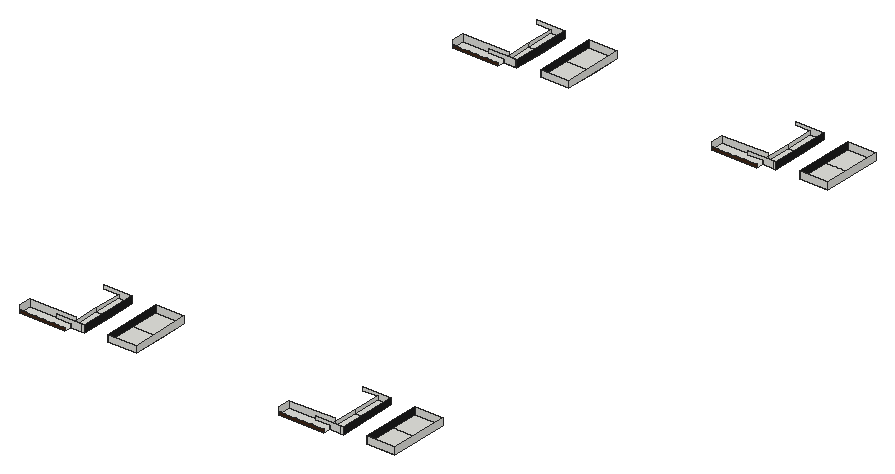
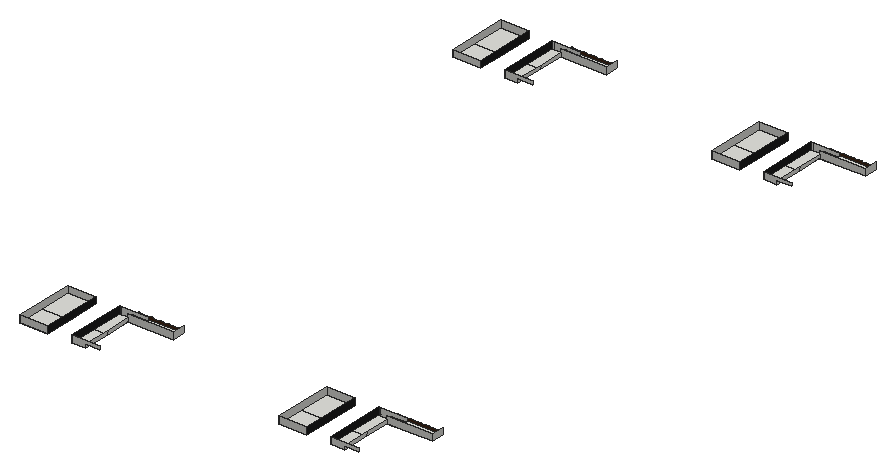
# SketchUp Ruby script. Lengths in inches.
U = 1.inch
M = Sketchup.active_model
def pt(a) = Geom::Point3d.new(a.map { |v| v * U })
def face(e, loops, mat)
  f = e.add_face(loops[0].map { |a| pt(a) })
  loops[1..].each { |l| e.add_face(l.map { |a| pt(a) }).erase! }
  f.material = f.back_material = mat if mat
  f
end
# faces: each face lists its corners as indices into pts; further lists are holes
def faces(e, pts, list, mat = nil) = list.each { |f| face(e, (f[0].is_a?(Array) ? f : [f]).map { |l| l.map { |i| pts[i] } }, mat) }
# xy, xz, yz: faces in a plane at the given z, y or x. An outline is a flat list of corners, or four numbers for a rectangle; further outlines are holes
def ring(l) = l.size == 4 ? [[l[0], l[1]], [l[2], l[1]], [l[2], l[3]], [l[0], l[3]]] : l.each_slice(2).to_a
def flat(e, list, mat, &to3) = list.each { |f| face(e, (f[0].is_a?(Array) ? f : [f]).map { |l| ring(l).map { |u, v| to3.(u, v) } }, mat) }
def xy(e, z, list, mat = nil) = flat(e, list, mat) { |x, y| [x, y, z] }
def xz(e, y, list, mat = nil) = flat(e, list, mat) { |x, z| [x, y, z] }
def yz(e, x, list, mat = nil) = flat(e, list, mat) { |y, z| [x, y, z] }
def lines(e, pts, list) = list.each { |a, b| e.add_line(pt(pts[a]), pt(pts[b])) }
# prism: a flat outline (further loops are holes) pulled along v
def prism(e, loops, v, mat = nil)
  f = face(e, loops, mat); d = Geom::Vector3d.new(v.map { |x| x * U })
  f.pushpull(f.normal.samedirection?(d) ? d.length : -d.length)
end
def box(e, o, s, mat = nil) = prism(e, [[o, [o[0] + s[0], o[1], o[2]], [o[0] + s[0], o[1] + s[1], o[2]], [o[0], o[1] + s[1], o[2]]]], [0, 0, s[2]], mat)
def at(x, y, z, deg = 0) = Geom::Transformation.translation(pt([x, y, z])) * Geom::Transformation.rotation(ORIGIN, Z_AXIS, deg.degrees)
def axes(o, x, y, z) = Geom::Transformation.new([*x, 0, *y, 0, *z, 0, *pt(o).to_a, 1])
def part(name) = M.definitions.add(name)
# library, detail: a bought-in or finely detailed component or shape, given as its bounding box
def library(name, o, s) = part(name).tap { |d| box(d.entities, o, s) }
def detail(e, o, s) = box(e.add_group.entities, o, s)
def put(e, d, t, mat = nil) = e.add_instance(d, t).tap { |i| i.material = mat if mat }
def group(e, t, mat = nil) = e.add_group.tap { |g| g.transformation = t; g.material = mat if mat }.entities
root = M.entities
M.materials.add("[Color M08]").color = [30, 30, 30]
M.materials.add("[Wood Veneer 01]").color = [66, 38, 20]
xy(root,230.89,[[252.78,566.68,406.85,611.02],[1131.53,566.68,1285.6,611.02],[252.78,2402.3,406.85,2446.65],[1131.53,2402.3,1285.6,2446.65]])
xy(root,231,[[406.85,589.83,453.7,697.21],[534.46,589.83,629.77,697.21],[1285.6,589.83,1332.45,697.21],[1413.21,589.83,1508.52,697.21],[406.85,697.21,453.7,792.52],
  [534.46,697.21,629.77,792.52],[1285.6,697.21,1332.45,792.52],[1413.21,697.21,1508.52,792.52],[406.85,2425.46,453.7,2532.83],[534.46,2425.46,629.77,2532.83],
  [1285.6,2425.46,1332.45,2532.83],[1413.21,2425.46,1508.52,2532.83],[406.85,2532.83,453.7,2628.15],[534.46,2532.83,629.77,2628.15],[1285.6,2532.83,1332.45,2628.15],
  [1413.21,2532.83,1508.52,2628.15]])
xz(root,566.68,[[252.78,230.89,406.85,230.89,406.85,240.89,405.02,240.1,404.46,239.96,403.9375,239.81,403.25,239.53,402.7,239.49,401.98,239.42,401.18,239.28,400.41,239.15,399.78,238.9,398.39,238.9,397.63,238.89,396.95,238.89,396.27,238.88,395.73,238.875,394.97,238.86,394.23,238.83,393.66,238.8,393.08,238.74,392.42,238.6,391.85,238.51,391.32,238.33,390.63,238.08,389.95,237.84,389.26,237.5625,388.66,237.47,387.98,237.4,387.25,237.42,386.68,237.45,386.09,237.51,385.49,237.59,384.95,237.71,384.12,238,383.41,238.33,382.86,238.57,382.36,238.86,381.84,238.96,381.15,239.02,380.47,239.125,379.73,239.04,379.16,238.66,378.57,238.61,377.91,238.55,377.39,238.27,376.71,238.18,376.03,238.18,375.36,238.11,374.83,238.15,374.01,238.19,373.4375,238.26,372.87,238.48,372.21,238.56,371.64,238.67,371.12,239.01,370.4375,239.18,369.8125,239.5,369.05,239.65,368.4375,239.8,367.68,239.96,367.03,240.23,366.45,240.27,365.8,240.43,365.23,240.43,364.65,240.42,364.125,240.41,363.43,240.4,362.74,240.37,362.05,240.33,361.37,240.27,360.69,240.17,360.07,239.97,359.42,239.75,358.68,239.375,357.89,239.08,357.01,238.72,356.26,238.46,355.04,238.14,353.92,237.88,353.27,237.87,352.4,237.74,351.69,237.79,350.92,237.86,350.29,238.15,349.52,238.19,348.9,238.25,348.14,238.45,347.45,238.62,342.56,238.62,342,238.625,341.14,238.625,340.45,238.63,339.83,238.64,339.05,238.65,338.38,238.66,337.69,238.6875,337.02,238.73,336.54,238.78,335.66,238.93,334.89,239.07,334.34,239.16,333.49,239.44,332.82,239.56,332.21,239.72,331.48,239.7,330.92,239.69,330.33,239.65,329.71,239.6,329.22,239.54,328.41,239.31,327.41,239.22,326.83,239.12,326.1875,238.76,325.55,238.51,324.99,238.375,324.55,238.02,323.85,237.74,323.23,237.43,322.38,237.22,321.7,236.98,321.09,237.01,320.4,237.04,319.64,237.11,318.95,237.2,318.42,237.33,317.75,237.68,316.8125,237.96,316.25,238.28,315.47,238.43,314.69,238.78,314.02,238.79,313.48,238.8,312.72,238.83,311.97,238.875,311.4,238.94,310.82,239.04,310.16,239.29,309.58,239.53,309.05,239.7,308.36,239.92,307.73,240.11,306.95,240.27,306.33,240.25,305.625,240.23,304.86,240.19,304.1875,240.12,303.53,240.03,302.89,239.85,302.34,239.52,301.78,239.35,301.19,239.18,300.68,238.86,299.99,238.72,299.17,238.59,298.66,238.34,293.09,238.34,292.41,238.33,291.18,238.33,290.46,238.32,289.61,238.3,288.98,238.28,288.23,238.26,287.6,238.15,286.84,238.13,286.29,238.1,285.4375,237.98,284.82,237.94,284.06,237.89,283.39,237.65,282.08,237.65,281.39,237.66,280.64,237.67,280.04,237.68,279.43,237.71,278.72,237.76,278.03,237.82,277.37,237.9,276.43,238.21,275.96,238.31,275.05,238.43,274.4,238.74,273.82,239.11,273.24,239.38,272.78,239.71,272.08,240.11,271.39,240.09,270.73,240.05,270.14,239.99,269.41,239.88,268.86,239.69,268.28,239.55,267.72,238.9375,267.19,238.77,266.45,238.79,265.58,238.8,265.07,238.82,264.03,238.92,263.34,238.93,262.64,238.94,261.94,238.97,261.26,239.03,260.57,239.09,259.79,239.19,259.28,239.52,258.72,239.64,258.27,239.86,257.48,240.2,256.88,240.59,256.34,240.85,255.32,241.55,254.05,241.69,252.84,241.52,252.78,241.52],[1131.53,230.89,1285.6,230.89,1285.6,240.89,1283.77,240.1,1283.21,239.96,1282.6875,239.81,1282,239.53,1281.45,239.49,1280.73,239.42,1279.93,239.28,1279.16,239.15,1278.53,238.9,1277.14,238.9,1276.38,238.89,1275.7,238.89,1275.02,238.88,1274.48,238.875,1273.72,238.86,1272.98,238.83,1272.41,238.8,1271.83,238.74,1271.17,238.6,1270.6,238.51,1270.07,238.33,1269.38,238.08,1268.7,237.84,1268.01,237.5625,1267.41,237.47,1266.73,237.4,1266,237.42,1265.43,237.45,1264.84,237.51,1264.24,237.59,1263.7,237.71,1262.87,238,1262.16,238.33,1261.61,238.57,1261.11,238.86,1260.59,238.96,1259.9,239.02,1259.22,239.125,1258.48,239.04,1257.91,238.66,1257.32,238.61,1256.66,238.55,1256.14,238.27,1255.46,238.18,1254.78,238.18,1254.11,238.11,1253.58,238.15,1252.76,238.19,1252.1875,238.26,1251.62,238.48,1250.96,238.56,1250.39,238.67,1249.87,239.01,1249.1875,239.18,1248.5625,239.5,1247.8,239.65,1247.1875,239.8,1246.43,239.96,1245.78,240.23,1245.2,240.27,1244.55,240.43,1243.98,240.43,1243.4,240.42,1242.875,240.41,1242.18,240.4,1241.49,240.37,1240.8,240.33,1240.12,240.27,1239.44,240.17,1238.82,239.97,1238.17,239.75,1237.43,239.375,1236.64,239.08,1235.76,238.72,1235.01,238.46,1233.79,238.14,1232.67,237.88,1232.02,237.87,1231.15,237.74,1230.44,237.79,1229.67,237.86,1229.04,238.15,1228.27,238.19,1227.65,238.25,1226.89,238.45,1226.2,238.62,1221.31,238.62,1220.75,238.625,1219.89,238.625,1219.2,238.63,1218.58,238.64,1217.8,238.65,1217.13,238.66,1216.44,238.6875,1215.77,238.73,1215.29,238.78,1214.41,238.93,1213.64,239.07,1213.09,239.16,1212.24,239.44,1211.57,239.56,1210.96,239.72,1210.23,239.7,1209.67,239.69,1209.08,239.65,1208.46,239.6,1207.97,239.54,1207.16,239.31,1206.16,239.22,1205.58,239.12,1204.9375,238.76,1204.3,238.51,1203.74,238.375,1203.3,238.02,1202.6,237.74,1201.98,237.43,1201.13,237.22,1200.45,236.98,1199.84,237.01,1199.15,237.04,1198.39,237.11,1197.7,237.2,1197.17,237.33,1196.5,237.68,1195.5625,237.96,1195,238.28,1194.22,238.43,1193.44,238.78,1192.77,238.79,1192.23,238.8,1191.47,238.83,1190.72,238.875,1190.15,238.94,1189.57,239.04,1188.91,239.29,1188.33,239.53,1187.8,239.7,1187.11,239.92,1186.48,240.11,1185.7,240.27,1185.08,240.25,1184.375,240.23,1183.61,240.19,1182.9375,240.12,1182.28,240.03,1181.64,239.85,1181.09,239.52,1180.53,239.35,1179.94,239.18,1179.43,238.86,1178.74,238.72,1177.92,238.59,1177.41,238.34,1171.84,238.34,1171.16,238.33,1169.93,238.33,1169.21,238.32,1168.36,238.3,1167.73,238.28,1166.98,238.26,1166.35,238.15,1165.59,238.13,1165.04,238.1,1164.1875,237.98,1163.57,237.94,1162.81,237.89,1162.14,237.65,1160.83,237.65,1160.14,237.66,1159.39,237.67,1158.79,237.68,1158.18,237.71,1157.47,237.76,1156.78,237.82,1156.12,237.9,1155.18,238.21,1154.71,238.31,1153.8,238.43,1153.15,238.74,1152.57,239.11,1151.99,239.38,1151.53,239.71,1150.83,240.11,1150.14,240.09,1149.48,240.05,1148.89,239.99,1148.16,239.88,1147.61,239.69,1147.03,239.55,1146.47,238.9375,1145.94,238.77,1145.2,238.79,1144.33,238.8,1143.82,238.82,1142.78,238.92,1142.09,238.93,1141.39,238.94,1140.69,238.97,1140.01,239.03,1139.32,239.09,1138.54,239.19,1138.03,239.52,1137.47,239.64,1137.02,239.86,1136.23,240.2,1135.63,240.59,1135.09,240.85,1134.07,241.55,1132.8,241.69,1131.59,241.52,1131.53,241.52]],"[Wood Veneer 01]")
xz(root,589.83,[[406.85,231,444.78,231,444.78,254.5,358.39,254.5,358.39,242.625,406.85,242.625],[444.78,231,453.7,254.5],[534.46,231,629.77,254.5],[1285.6,231,1323.53,231,1323.53,254.5,1237.14,254.5,1237.14,242.625,1285.6,242.625],[1323.53,231,1332.45,254.5],
  [1413.21,231,1508.52,254.5]])
xz(root,611.02,[[252.78,230.89,406.85,254.5],[1131.53,230.89,1285.6,254.5]])
xz(root,792.52,[[406.85,231,406.85,242.625,358.39,242.625,358.39,254.5,453.7,254.5,453.7,231],[534.46,231,629.77,254.5],[1285.6,231,1285.6,242.625,1237.14,242.625,1237.14,254.5,1332.45,254.5,1332.45,231],[1413.21,231,1508.52,254.5]])
xz(root,2402.3,[[252.78,230.89,406.85,230.89,406.85,240.89,405.02,240.1,404.46,239.96,403.9375,239.81,403.25,239.53,402.7,239.49,401.98,239.42,401.18,239.28,400.41,239.15,399.78,238.9,398.39,238.9,397.63,238.89,396.95,238.89,396.27,238.88,395.73,238.875,394.97,238.86,394.23,238.83,393.66,238.8,393.08,238.74,392.42,238.6,391.85,238.51,391.32,238.33,390.63,238.08,389.95,237.84,389.26,237.5625,388.66,237.47,387.98,237.4,387.25,237.42,386.68,237.45,386.09,237.51,385.49,237.59,384.95,237.71,384.12,238,383.41,238.33,382.86,238.57,382.36,238.86,381.84,238.96,381.15,239.02,380.47,239.125,379.73,239.04,379.16,238.66,378.57,238.61,377.91,238.55,377.39,238.27,376.71,238.18,376.03,238.18,375.36,238.11,374.83,238.15,374.01,238.19,373.4375,238.26,372.87,238.48,372.21,238.56,371.64,238.67,371.12,239.01,370.4375,239.18,369.8125,239.5,369.05,239.65,368.4375,239.8,367.68,239.96,367.03,240.23,366.45,240.27,365.8,240.43,365.23,240.43,364.65,240.42,364.125,240.41,363.43,240.4,362.74,240.37,362.05,240.33,361.37,240.27,360.69,240.17,360.07,239.97,359.42,239.75,358.68,239.375,357.89,239.08,357.01,238.72,356.26,238.46,355.04,238.14,353.92,237.88,353.27,237.87,352.4,237.74,351.69,237.79,350.92,237.86,350.29,238.15,349.52,238.19,348.9,238.25,348.14,238.45,347.45,238.62,342.56,238.62,342,238.625,341.14,238.625,340.45,238.63,339.83,238.64,339.05,238.65,338.38,238.66,337.69,238.6875,337.02,238.73,336.54,238.78,335.66,238.93,334.89,239.07,334.34,239.16,333.49,239.44,332.82,239.56,332.21,239.72,331.48,239.7,330.92,239.69,330.33,239.65,329.71,239.6,329.22,239.54,328.41,239.31,327.41,239.22,326.83,239.12,326.1875,238.76,325.55,238.51,324.99,238.375,324.55,238.02,323.85,237.74,323.23,237.43,322.38,237.22,321.7,236.98,321.09,237.01,320.4,237.04,319.64,237.11,318.95,237.2,318.42,237.33,317.75,237.68,316.8125,237.96,316.25,238.28,315.47,238.43,314.69,238.78,314.02,238.79,313.48,238.8,312.72,238.83,311.97,238.875,311.4,238.94,310.82,239.04,310.16,239.29,309.58,239.53,309.05,239.7,308.36,239.92,307.73,240.11,306.95,240.27,306.33,240.25,305.625,240.23,304.86,240.19,304.1875,240.12,303.53,240.03,302.89,239.85,302.34,239.52,301.78,239.35,301.19,239.18,300.68,238.86,299.99,238.72,299.17,238.59,298.66,238.34,293.09,238.34,292.41,238.33,291.18,238.33,290.46,238.32,289.61,238.3,288.98,238.28,288.23,238.26,287.6,238.15,286.84,238.13,286.29,238.1,285.4375,237.98,284.82,237.94,284.06,237.89,283.39,237.65,282.08,237.65,281.39,237.66,280.64,237.67,280.04,237.68,279.43,237.71,278.72,237.76,278.03,237.82,277.37,237.9,276.43,238.21,275.96,238.31,275.05,238.43,274.4,238.74,273.82,239.11,273.24,239.38,272.78,239.71,272.08,240.11,271.39,240.09,270.73,240.05,270.14,239.99,269.41,239.88,268.86,239.69,268.28,239.55,267.72,238.9375,267.19,238.77,266.45,238.79,265.58,238.8,265.07,238.82,264.03,238.92,263.34,238.93,262.64,238.94,261.94,238.97,261.26,239.03,260.57,239.09,259.79,239.19,259.28,239.52,258.72,239.64,258.27,239.86,257.48,240.2,256.88,240.59,256.34,240.85,255.32,241.55,254.05,241.69,252.84,241.52,252.78,241.52],[1131.53,230.89,1285.6,230.89,1285.6,240.89,1283.77,240.1,1283.21,239.96,1282.6875,239.81,1282,239.53,1281.45,239.49,1280.73,239.42,1279.93,239.28,1279.16,239.15,1278.53,238.9,1277.14,238.9,1276.38,238.89,1275.7,238.89,1275.02,238.88,1274.48,238.875,1273.72,238.86,1272.98,238.83,1272.41,238.8,1271.83,238.74,1271.17,238.6,1270.6,238.51,1270.07,238.33,1269.38,238.08,1268.7,237.84,1268.01,237.5625,1267.41,237.47,1266.73,237.4,1266,237.42,1265.43,237.45,1264.84,237.51,1264.24,237.59,1263.7,237.71,1262.87,238,1262.16,238.33,1261.61,238.57,1261.11,238.86,1260.59,238.96,1259.9,239.02,1259.22,239.125,1258.48,239.04,1257.91,238.66,1257.32,238.61,1256.66,238.55,1256.14,238.27,1255.46,238.18,1254.78,238.18,1254.11,238.11,1253.58,238.15,1252.76,238.19,1252.1875,238.26,1251.62,238.48,1250.96,238.56,1250.39,238.67,1249.87,239.01,1249.1875,239.18,1248.5625,239.5,1247.8,239.65,1247.1875,239.8,1246.43,239.96,1245.78,240.23,1245.2,240.27,1244.55,240.43,1243.98,240.43,1243.4,240.42,1242.875,240.41,1242.18,240.4,1241.49,240.37,1240.8,240.33,1240.12,240.27,1239.44,240.17,1238.82,239.97,1238.17,239.75,1237.43,239.375,1236.64,239.08,1235.76,238.72,1235.01,238.46,1233.79,238.14,1232.67,237.88,1232.02,237.87,1231.15,237.74,1230.44,237.79,1229.67,237.86,1229.04,238.15,1228.27,238.19,1227.65,238.25,1226.89,238.45,1226.2,238.62,1221.31,238.62,1220.75,238.625,1219.89,238.625,1219.2,238.63,1218.58,238.64,1217.8,238.65,1217.13,238.66,1216.44,238.6875,1215.77,238.73,1215.29,238.78,1214.41,238.93,1213.64,239.07,1213.09,239.16,1212.24,239.44,1211.57,239.56,1210.96,239.72,1210.23,239.7,1209.67,239.69,1209.08,239.65,1208.46,239.6,1207.97,239.54,1207.16,239.31,1206.16,239.22,1205.58,239.12,1204.9375,238.76,1204.3,238.51,1203.74,238.375,1203.3,238.02,1202.6,237.74,1201.98,237.43,1201.13,237.22,1200.45,236.98,1199.84,237.01,1199.15,237.04,1198.39,237.11,1197.7,237.2,1197.17,237.33,1196.5,237.68,1195.5625,237.96,1195,238.28,1194.22,238.43,1193.44,238.78,1192.77,238.79,1192.23,238.8,1191.47,238.83,1190.72,238.875,1190.15,238.94,1189.57,239.04,1188.91,239.29,1188.33,239.53,1187.8,239.7,1187.11,239.92,1186.48,240.11,1185.7,240.27,1185.08,240.25,1184.375,240.23,1183.61,240.19,1182.9375,240.12,1182.28,240.03,1181.64,239.85,1181.09,239.52,1180.53,239.35,1179.94,239.18,1179.43,238.86,1178.74,238.72,1177.92,238.59,1177.41,238.34,1171.84,238.34,1171.16,238.33,1169.93,238.33,1169.21,238.32,1168.36,238.3,1167.73,238.28,1166.98,238.26,1166.35,238.15,1165.59,238.13,1165.04,238.1,1164.1875,237.98,1163.57,237.94,1162.81,237.89,1162.14,237.65,1160.83,237.65,1160.14,237.66,1159.39,237.67,1158.79,237.68,1158.18,237.71,1157.47,237.76,1156.78,237.82,1156.12,237.9,1155.18,238.21,1154.71,238.31,1153.8,238.43,1153.15,238.74,1152.57,239.11,1151.99,239.38,1151.53,239.71,1150.83,240.11,1150.14,240.09,1149.48,240.05,1148.89,239.99,1148.16,239.88,1147.61,239.69,1147.03,239.55,1146.47,238.9375,1145.94,238.77,1145.2,238.79,1144.33,238.8,1143.82,238.82,1142.78,238.92,1142.09,238.93,1141.39,238.94,1140.69,238.97,1140.01,239.03,1139.32,239.09,1138.54,239.19,1138.03,239.52,1137.47,239.64,1137.02,239.86,1136.23,240.2,1135.63,240.59,1135.09,240.85,1134.07,241.55,1132.8,241.69,1131.59,241.52,1131.53,241.52]],"[Wood Veneer 01]")
xz(root,2425.46,[[406.85,231,444.78,231,444.78,254.5,358.39,254.5,358.39,242.625,406.85,242.625],[444.78,231,453.7,254.5],[534.46,231,629.77,254.5],[1285.6,231,1323.53,231,1323.53,254.5,1237.14,254.5,1237.14,242.625,1285.6,242.625],[1323.53,231,1332.45,254.5],
  [1413.21,231,1508.52,254.5]])
xz(root,2446.65,[[252.78,230.89,406.85,254.5],[1131.53,230.89,1285.6,254.5]])
xz(root,2628.15,[[406.85,231,406.85,242.625,358.39,242.625,358.39,254.5,453.7,254.5,453.7,231],[534.46,231,629.77,254.5],[1285.6,231,1285.6,242.625,1237.14,242.625,1237.14,254.5,1332.45,254.5,1332.45,231],[1413.21,231,1508.52,254.5]])
yz(root,252.78,[[566.68,230.89,566.68,241.52,568.68,241.52,568.68,254.5,611.02,254.5,611.02,230.89],[2402.3,230.89,2402.3,241.52,2404.3,241.52,2404.3,254.5,2446.65,254.5,2446.65,230.89]])
yz(root,406.85,[[589.83,230.89,611.02,231],[2425.46,230.89,2446.65,231],[589.83,231,611.02,242.625],[611.02,231,697.21,242.625],[697.21,231,792.52,242.625],
  [2425.46,231,2446.65,242.625],[2446.65,231,2532.83,242.625],[2532.83,231,2628.15,242.625]])
yz(root,453.7,[[589.83,231,792.52,254.5],[2425.46,231,2628.15,254.5]],"[Color M08]")
yz(root,534.46,[[589.83,231,792.52,254.5],[2425.46,231,2628.15,254.5]],"[Color M08]")
yz(root,629.77,[[589.83,231,792.52,254.5],[2425.46,231,2628.15,254.5]])
yz(root,1131.53,[[566.68,230.89,566.68,241.52,568.68,241.52,568.68,254.5,611.02,254.5,611.02,230.89],[2402.3,230.89,2402.3,241.52,2404.3,241.52,2404.3,254.5,2446.65,254.5,2446.65,230.89]])
yz(root,1285.6,[[589.83,230.89,611.02,231],[2425.46,230.89,2446.65,231],[589.83,231,611.02,242.625],[611.02,231,697.21,242.625],[697.21,231,792.52,242.625],
  [2425.46,231,2446.65,242.625],[2446.65,231,2532.83,242.625],[2532.83,231,2628.15,242.625]])
yz(root,1332.45,[[589.83,231,792.52,254.5],[2425.46,231,2628.15,254.5]],"[Color M08]")
yz(root,1413.21,[[589.83,231,792.52,254.5],[2425.46,231,2628.15,254.5]],"[Color M08]")
yz(root,1508.52,[[589.83,231,792.52,254.5],[2425.46,231,2628.15,254.5]])
